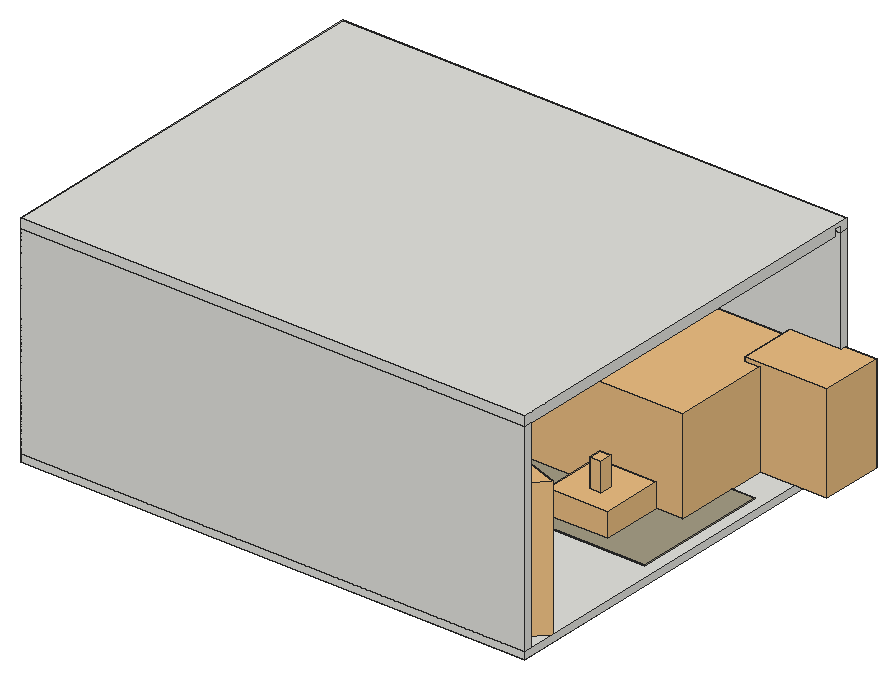
# SketchUp Ruby script. Lengths in inches.
U = 1.inch
M = Sketchup.active_model
def pt(a) = Geom::Point3d.new(a.map { |v| v * U })
def face(e, loops, mat)
  f = e.add_face(loops[0].map { |a| pt(a) })
  loops[1..].each { |l| e.add_face(l.map { |a| pt(a) }).erase! }
  f.material = f.back_material = mat if mat
  f
end
# faces: each face lists its corners as indices into pts; further lists are holes
def faces(e, pts, list, mat = nil) = list.each { |f| face(e, (f[0].is_a?(Array) ? f : [f]).map { |l| l.map { |i| pts[i] } }, mat) }
# xy, xz, yz: faces in a plane at the given z, y or x. An outline is a flat list of corners, or four numbers for a rectangle; further outlines are holes
def ring(l) = l.size == 4 ? [[l[0], l[1]], [l[2], l[1]], [l[2], l[3]], [l[0], l[3]]] : l.each_slice(2).to_a
def flat(e, list, mat, &to3) = list.each { |f| face(e, (f[0].is_a?(Array) ? f : [f]).map { |l| ring(l).map { |u, v| to3.(u, v) } }, mat) }
def xy(e, z, list, mat = nil) = flat(e, list, mat) { |x, y| [x, y, z] }
def xz(e, y, list, mat = nil) = flat(e, list, mat) { |x, z| [x, y, z] }
def yz(e, x, list, mat = nil) = flat(e, list, mat) { |y, z| [x, y, z] }
def lines(e, pts, list) = list.each { |a, b| e.add_line(pt(pts[a]), pt(pts[b])) }
# prism: a flat outline (further loops are holes) pulled along v
def prism(e, loops, v, mat = nil)
  f = face(e, loops, mat); d = Geom::Vector3d.new(v.map { |x| x * U })
  f.pushpull(f.normal.samedirection?(d) ? d.length : -d.length)
end
def box(e, o, s, mat = nil) = prism(e, [[o, [o[0] + s[0], o[1], o[2]], [o[0] + s[0], o[1] + s[1], o[2]], [o[0], o[1] + s[1], o[2]]]], [0, 0, s[2]], mat)
def at(x, y, z, deg = 0) = Geom::Transformation.translation(pt([x, y, z])) * Geom::Transformation.rotation(ORIGIN, Z_AXIS, deg.degrees)
def axes(o, x, y, z) = Geom::Transformation.new([*x, 0, *y, 0, *z, 0, *pt(o).to_a, 1])
def part(name) = M.definitions.add(name)
# library, detail: a bought-in or finely detailed component or shape, given as its bounding box
def library(name, o, s) = part(name).tap { |d| box(d.entities, o, s) }
def detail(e, o, s) = box(e.add_group.entities, o, s)
def put(e, d, t, mat = nil) = e.add_instance(d, t).tap { |i| i.material = mat if mat }
def group(e, t, mat = nil) = e.add_group.tap { |g| g.transformation = t; g.material = mat if mat }.entities
root = M.entities
M.materials.add("Carpet").color = [165, 157, 133]
M.materials.add("Glazing").color = [128, 128, 128]
M.materials["Glazing"].alpha = 0.05
M.materials.add("Powdercoating").color = [41, 44, 40]
c1 = part("Group\#15")
xy(c1.entities,0,[[0,-55.94,0.71,45.94]])
xy(c1.entities,0.2,[[0,-55.94,0.47,45.94],[0.47,45.94,0.71,46.42]])
xy(c1.entities,2.36,[[0.47,-55.94,0.71,46.42]])
xz(c1.entities,-55.94,[[0,0,0.71,0,0.71,2.36,0.47,2.36,0.47,0.2,0,0.2]])
xz(c1.entities,45.94,[[0,0,0.71,0.2]])
xz(c1.entities,46.42,[[0.47,0.2,0.71,2.36]])
yz(c1.entities,0,[[-55.94,0,45.94,0.2]])
yz(c1.entities,0.47,[[-55.94,0.2,46.42,2.36]])
yz(c1.entities,0.71,[[-55.94,0,45.94,0,45.94,0.2,46.42,0.2,46.42,2.36,-55.94,2.36]])
c2 = part("Group\#11")
xy(c2.entities,0,[[0,-59.09,0.71,45.94]])
xy(c2.entities,0.2,[[0,-59.09,0.47,45.94],[0.47,45.94,0.71,46.42]])
xy(c2.entities,2.36,[[0.47,-59.09,0.71,46.42]])
xz(c2.entities,-59.09,[[0,0,0.71,0,0.71,2.36,0.47,2.36,0.47,0.2,0,0.2]])
xz(c2.entities,45.94,[[0,0,0.71,0.2]])
xz(c2.entities,46.42,[[0.47,0.2,0.71,2.36]])
yz(c2.entities,0,[[-59.09,0,45.94,0.2]])
yz(c2.entities,0.47,[[-59.09,0.2,46.42,2.36]])
yz(c2.entities,0.71,[[-59.09,0,45.94,0,45.94,0.2,46.42,0.2,46.42,2.36,-59.09,2.36]])
c3 = part("Group\#16")
prism(c3.entities,[[[0.47,-56.18,0.2],[0,-56.18,0.2],[0,-56.18,0],[0.71,-56.18,0],[0.71,-56.18,2.36],[0.47,-56.18,2.36]]],[0,28.68,0])
c4 = part("Group\#12")
box(c4.entities,[-0.73,0,0],[27.99,0.55,102.05])
c5 = part("Group\#18")
xy(c5.entities,0,[[0.47,-56.18,0.47,-55.47,0,-55.47,0,-28.21,1.18,-28.21,1.18,-56.18]])
xy(c5.entities,0.2,[[0.71,-56.18,1.18,-28.21],[0,-55.47,0.47,-28.21],[0.47,-28.21,0.71,-27.74]])
xy(c5.entities,2.36,[[0.47,-56.18,0.71,-27.74]])
xz(c5.entities,-56.18,[[0.47,0,1.18,0,1.18,0.2,0.71,0.2,0.71,2.36,0.47,2.36]])
xz(c5.entities,-55.47,[[0,0,0.47,0.2]])
xz(c5.entities,-28.21,[[0,0,1.18,0.2]])
xz(c5.entities,-27.74,[[0.47,0.2,0.71,2.36]])
yz(c5.entities,0,[[-55.47,0,-28.21,0.2]])
yz(c5.entities,0.47,[[-56.18,0,-55.47,0.2],[-56.18,0.2,-27.74,2.36]])
yz(c5.entities,0.71,[[-56.18,0.2,-27.74,2.36]])
yz(c5.entities,1.18,[[-56.18,0,-28.21,0.2]])
c6 = part("Group\#34")
xy(c6.entities,0,[[-20.45,0,7.76,1.22]])
xy(c6.entities,0.06,[[-20.39,0.06,7.7,1.22]])
xy(c6.entities,0.47,[[-19.98,0,7.28,0.06]])
xy(c6.entities,101.89,[[-19.98,0,7.28,0.06]])
xy(c6.entities,102.3,[[-20.39,0.06,7.7,1.22]])
xy(c6.entities,102.36,[[-20.45,0,7.76,1.22]])
xz(c6.entities,0,[[[-20.45,0,7.76,102.36],[-19.98,0.47,7.28,101.89]]])
xz(c6.entities,0.06,[[[-20.39,0.06,7.7,102.3],[-19.98,0.47,7.28,101.89]]])
xz(c6.entities,1.22,[[[-20.45,0,7.76,102.36],[-20.39,0.06,7.7,102.3]]])
yz(c6.entities,-20.45,[[0,0,1.22,102.36]])
yz(c6.entities,-20.39,[[0.06,0.06,1.22,102.3]])
yz(c6.entities,-19.98,[[0,0.47,0.06,101.89]])
yz(c6.entities,7.28,[[0,0.47,0.06,101.89]])
yz(c6.entities,7.7,[[0.06,0.06,1.22,102.3]])
yz(c6.entities,7.76,[[0,0,1.22,102.36]])
c7 = part("Group\#14")
put(c7.entities,c1,axes([27.97,0,7.875],[1,0,0],[0,0,-1],[0,1,0]),"Powdercoating")
put(c7.entities,c2,axes([0.71,0,6.8],[-1,0,0],[0,0,-0.97687],[0,1,0]),"Powdercoating")
put(c7.entities,c3,axes([-27.5,0,-38.07],[0,0,-1],[-1,0,0],[0,1,0]),"Powdercoating")
put(c7.entities,c4,at(1.12,0.35,-38.39),"Glazing")
put(c7.entities,c5,axes([-27.5,0,63.35],[0,0,1],[-1,0,0],[0,1,0]),"Powdercoating")
put(c7.entities,c6,at(20.6875,1.0625,-38.54),"Powdercoating")
c8 = part("Sliding door panels")
put(c8.entities,c7,at(-1.18,4.5,38.86))
g1 = group(c8.entities,at(84.74,4.5,38.86))
put(g1,c1,axes([-27.97,0,7.875],[-1,0,0],[0,0,-1],[0,1,0]),"Powdercoating")
put(g1,c2,axes([-0.71,0,6.8],[1,0,0],[0,0,-0.97687],[0,1,0]),"Powdercoating")
put(g1,c3,axes([27.5,0,-38.07],[0,0,-1],[1,0,0],[0,1,0]),"Powdercoating")
put(g1,c4,axes([-1.12,0.35,-38.39],[-1,0,0],[0,1,0],[0,0,1]),"Glazing")
put(g1,c5,axes([27.5,0,63.35],[0,0,1],[1,0,0],[0,1,0]),"Powdercoating")
put(g1,c6,axes([-20.6875,1.0625,-38.54],[-1,0,0],[0,1,0],[0,0,1]),"Powdercoating")
g2 = group(c8.entities,at(56.0625,4.5,38.86))
put(g2,c1,axes([-27.97,0,7.875],[-1,0,0],[0,0,-1],[0,1,0]),"Powdercoating")
put(g2,c3,axes([27.5,0,-38.07],[0,0,-1],[1,0,0],[0,1,0]),"Powdercoating")
put(g2,c4,axes([-1.12,0.35,-38.39],[-1,0,0],[0,1,0],[0,0,1]),"Glazing")
put(g2,c5,axes([27.5,0,63.35],[0,0,1],[1,0,0],[0,1,0]),"Powdercoating")
put(g2,c6,axes([-20.6875,1.0625,-38.54],[-1,0,0],[0,1,0],[0,0,1]),"Powdercoating")
g3 = group(g2,at(-0.71,0,6.8),"Powdercoating")
xy(g3,-45.34,[[0.47,0.2,0.71,2.36]])
xy(g3,-44.88,[[0,0,0.71,0.2]])
xy(g3,57.73,[[0,0,0.71,0,0.71,2.36,0.47,2.36,0.47,0.2,0,0.2]])
xz(g3,0,[[0,-44.88,0.71,57.73]])
xz(g3,0.2,[[0.47,-45.34,0.71,-44.88],[0,-44.88,0.47,57.73]])
xz(g3,2.36,[[0.47,-45.34,0.71,57.73]])
yz(g3,0,[[0,-44.88,0.2,57.73]])
yz(g3,0.47,[[0.2,-45.34,2.36,57.73]])
yz(g3,0.71,[[0.2,-45.34,2.36,-45.34,2.36,57.73,0,57.73,0,-44.88,0.2,-44.88]])
put(c8.entities,c7,axes([-33.94,4.5,38.86],[1.14218,0,0],[0,1,0],[0,0,1]))
c9 = part("sliding door")
put(c9.entities,c8,at(0,-4.5,-0.08))
c10 = library("____",[-857.35,-17.89,-0.54],[1669.93,232.85,2261.28])
c11 = library("_________4",[391.51,-229.42,0.9375],[996.96,302.79,2265.625])
c12 = library("_________5\#1",[-1361.6,-221.02,-25.09],[914.12,296.77,2295.03])
c13 = library("door58",[0,0,0],[34.0625,4.69,78.29])
c14 = library("Sectional sofa",[-0.93,-10.63,-23.92],[126.92,88.46,78.25])
c15 = part("Vertical bar")
box(c15.entities,[0,0,0],[0.875,0.8,31.5])
c16 = library("skpE45D",[-24.47,-26.97,0],[48.94,53.94,77.79])
c17 = part("Tapete")
box(c17.entities,[0,0,0],[73.55,109.57,0.42],"Carpet")
c18 = part("02 Tapete")
put(c18.entities,c17,at(0.05,-109.34,0))
c19 = part("Carpet")
put(c19.entities,c18,at(0,0,0))
c20 = library("Round Coffe Table",[-17.98,-18.01,-0.01],[35.96,36.02,14.19])
c21 = library("191418",[-24.78,-19.8125,0],[49.1,36.6,58.24])
c22 = library("Flower Vase",[5.42,3.34,0],[6.62,7.58,17.36])
c23 = part("Component\#6")
xy(c23.entities,0,[[[1.86,0,1.34,0.1,0.88,0.34,0.49,0.68,0.2,1.12,0.03,1.61,0,2.13,0.1,2.65,0.34,3.11,0.68,3.5,1.12,3.79,1.61,3.96,2.13,3.99,2.65,3.89,3.11,3.65,3.5,3.31,3.79,2.87,3.96,2.38,3.99,1.86,3.89,1.34,3.65,0.88,3.31,0.49,2.87,0.2,2.38,0.03],[1.9,0.61,2.26,0.64,2.6,0.75,2.9,0.95,3.14,1.22,3.3,1.54,3.375,1.9,3.35,2.26,3.24,2.6,3.04,2.9,2.77,3.14,2.45,3.3,2.09,3.375,1.73,3.35,1.39,3.24,1.09,3.04,0.85,2.77,0.6875,2.45,0.61,2.09,0.64,1.73,0.75,1.39,0.95,1.09,1.22,0.85,1.54,0.6875]]])
xy(c23.entities,0.125,[[1.9,0.61,1.54,0.6875,1.22,0.85,0.95,1.09,0.75,1.39,0.64,1.73,0.61,2.09,0.6875,2.45,0.85,2.77,1.09,3.04,1.39,3.24,1.73,3.35,2.09,3.375,2.45,3.3,2.77,3.14,3.04,2.9,3.24,2.6,3.35,2.26,3.375,1.9,3.3,1.54,3.14,1.22,2.9,0.95,2.6,0.75,2.26,0.64]])
xy(c23.entities,0.75,[[1.86,0,2.38,0.03,2.87,0.2,3.31,0.49,3.65,0.88,3.89,1.34,3.99,1.86,3.96,2.38,3.79,2.87,3.5,3.31,3.11,3.65,2.65,3.89,2.13,3.99,1.61,3.96,1.12,3.79,0.68,3.5,0.34,3.11,0.1,2.65,0,2.13,0.03,1.61,0.2,1.12,0.49,0.68,0.88,0.34,1.34,0.1]])
p = [[1.34,0.1,0],[1.86,0,0],[1.86,0,0.75],[1.34,0.1,0.75],[2.38,0.03,0],[2.38,0.03,0.75],
  [2.87,0.2,0],[2.87,0.2,0.75],[0.88,0.34,0],[0.88,0.34,0.75],[3.31,0.49,0],[3.31,0.49,0.75],
  [0.49,0.68,0],[0.49,0.68,0.75],[3.65,0.88,0],[3.65,0.88,0.75],[1.9,0.61,0],[1.54,0.6875,0],
  [1.54,0.6875,0.125],[1.9,0.61,0.125],[2.26,0.64,0],[2.26,0.64,0.125],[2.6,0.75,0],[2.6,0.75,0.125],
  [0.2,1.12,0],[0.2,1.12,0.75],[1.22,0.85,0],[1.22,0.85,0.125],[0.95,1.09,0],[0.95,1.09,0.125],
  [2.9,0.95,0],[2.9,0.95,0.125],[3.89,1.34,0],[3.89,1.34,0.75],[3.14,1.22,0],[3.14,1.22,0.125],
  [0.03,1.61,0],[0.03,1.61,0.75],[0.75,1.39,0],[0.75,1.39,0.125],[3.3,1.54,0],[3.3,1.54,0.125],
  [3.99,1.86,0],[3.99,1.86,0.75],[0.64,1.73,0],[0.64,1.73,0.125],[3.375,1.9,0],[3.375,1.9,0.125],
  [0,2.13,0],[0,2.13,0.75],[0.61,2.09,0],[0.61,2.09,0.125],[3.35,2.26,0],[3.35,2.26,0.125],
  [3.96,2.38,0],[3.96,2.38,0.75],[0.1,2.65,0],[0.1,2.65,0.75],[0.6875,2.45,0],[0.6875,2.45,0.125],
  [3.24,2.6,0],[3.24,2.6,0.125],[0.85,2.77,0],[0.85,2.77,0.125],[3.79,2.87,0],[3.79,2.87,0.75],
  [0.34,3.11,0],[0.34,3.11,0.75],[3.04,2.9,0],[3.04,2.9,0.125],[1.09,3.04,0],[1.09,3.04,0.125],
  [2.77,3.14,0],[2.77,3.14,0.125],[3.5,3.31,0],[3.5,3.31,0.75],[1.39,3.24,0],[1.39,3.24,0.125],
  [0.68,3.5,0],[0.68,3.5,0.75],[2.45,3.3,0],[2.45,3.3,0.125],[1.73,3.35,0],[1.73,3.35,0.125],
  [2.09,3.375,0],[2.09,3.375,0.125],[3.11,3.65,0],[3.11,3.65,0.75],[1.12,3.79,0],[1.12,3.79,0.75],
  [2.65,3.89,0],[2.65,3.89,0.75],[1.61,3.96,0],[1.61,3.96,0.75],[2.13,3.99,0],[2.13,3.99,0.75]]
faces(c23.entities,p,[[0,1,2,3],[1,4,5,2],[4,6,7,5],[8,0,3,9],[6,10,11,7],[12,8,9,13],[10,14,15,11],[16,17,18,19],
  [20,16,19,21],[22,20,21,23],[24,12,13,25],[17,26,27,18],[26,28,29,27],[30,22,23,31],[14,32,33,15],[34,30,31,35],
  [36,24,25,37],[28,38,39,29],[40,34,35,41],[32,42,43,33],[38,44,45,39],[46,40,41,47],[48,36,37,49],[44,50,51,45],
  [52,46,47,53],[42,54,55,43],[56,48,49,57],[50,58,59,51],[60,52,53,61],[58,62,63,59],[54,64,65,55],[66,56,57,67],
  [68,60,61,69],[62,70,71,63],[72,68,69,73],[64,74,75,65],[70,76,77,71],[78,66,67,79],[80,72,73,81],[76,82,83,77],
  [84,80,81,85],[74,86,87,75],[82,84,85,83],[88,78,79,89],[86,90,91,87],[92,88,89,93],[90,94,95,91],[94,92,93,95]])
c24 = library("VASE ",[-5.43,-0.85,0],[32.15,30.91,75.86])
c25 = part("Group30\#1")
p = [[30,30,37],[124.5,30,37],[30,115.5,37]]
lines(c25.entities,p,[[0,1],[0,2]])
c26 = part("Group29\#1")
put(c26.entities,c25,at(0,0,0))
c27 = part("Group\#40")
box(c27.entities,[0,0,87.15],[0.75,23.85,29.85])
xy(c27.entities,0,[[0,0,0.75,23.85]])
xy(c27.entities,14.11,[[0.25,0.25,0.75,23.6]])
xy(c27.entities,14.61,[[0.25,0.25,0.75,23.6]])
xy(c27.entities,14.86,[[0,0,0.75,23.85]])
xy(c27.entities,15.16,[[0,0,0.75,23.85]])
xy(c27.entities,29.26,[[0.25,0.25,0.75,23.6]])
xy(c27.entities,29.76,[[0.25,0.25,0.75,23.6]])
xy(c27.entities,30.01,[[0,0,0.75,23.85]])
xy(c27.entities,30.3125,[[0,0,0.75,23.85]])
xy(c27.entities,86.85,[[0,0,0.75,23.85]])
xz(c27.entities,0,[[0,0,0.75,14.86],[0,15.16,0.75,30.01],[0,30.3125,0.75,86.85]])
xz(c27.entities,0.25,[[0.25,14.11,0.75,14.61],[0.25,29.26,0.75,29.76]])
xz(c27.entities,23.6,[[0.25,14.11,0.75,14.61],[0.25,29.26,0.75,29.76]])
xz(c27.entities,23.85,[[0,0,0.75,14.86],[0,15.16,0.75,30.01],[0,30.3125,0.75,86.85]])
yz(c27.entities,0,[[0,0,23.85,14.86],[0,14.86,23.85,15.16],[0,15.16,23.85,30.01],[0,30.01,23.85,30.3125],[0,30.3125,23.85,86.85]])
yz(c27.entities,0.25,[[0.25,14.11,23.6,14.61],[0.25,29.26,23.6,29.76]])
yz(c27.entities,0.75,[[0,0,23.85,13.86],[[0,13.86,23.85,14.86],[0.25,14.11,23.6,14.61]],[0,15.16,23.85,29.01],[[0,29.01,23.85,30.01],[0.25,29.26,23.6,29.76]],[0,30.3125,23.85,86.85]])
p = [[0,0,86.85],[0,0,87.15],[0,23.85,86.85],[0,23.85,87.15]]
lines(c27.entities,p,[[0,1],[2,3]])
c28 = library("Agrupar\#9",[0,0,0],[23.62,23.23,23.62])
c29 = library("Group\#41",[0,0,-0.5],[89.46,0.75,39.5])
c30 = library("Group\#39",[0,0,0],[23.23,23.62,41.34])
c31 = library("Group\#38",[0,0,-0.5],[59.03,0.75,39.5])
c32 = library("Group\#45",[0,0,0],[67.25,19.4,51.93])
c33 = library("Groupe\#5",[0,0,0],[91.34,77.95,241.79])
c34 = library("Group\#46",[0,0,0],[2,2,36.3125])
p = [[17,36.7,61],[17,56.25,61],[17,76.1,61],[17,95.8,61]]
lines(root,p,[[0,1],[1,2],[2,3]])
put(root,c9,axes([69.57,235.5,4],[1.21,0,0],[0,1.4525,0],[0,0,1.04543]))
put(root,c10,axes([33.86,232,4.15],[0.01804,0,0],[0,0.02091,0],[0,0,0.05412]))
put(root,c11,axes([140.46,233.33,5.36],[0.03072,0,0],[0,0.01858,0],[0,0,0.05359]))
put(root,c12,axes([29.18,233.52,5.36],[0.01813,0,0],[0,0.01598,0],[0,0,0.05359]))
put(root,c10,axes([149.23,232,4.15],[0.01263,0,0],[0,0.02091,0],[0,0,0.05412]))
put(root,c13,axes([0,229.5,4],[0,-1.233,0],[1.05479,0,0],[0,0,1.07289]))
put(root,c14,at(277.88,222.27,5.63,-180))
put(root,c15,at(106,90,4))
put(root,c15,at(106,91.1875,4))
put(root,c15,at(106,92.38,4))
put(root,c15,at(106,93.57,4))
put(root,c15,at(106,94.76,4))
put(root,c15,at(106,95.95,4))
put(root,c15,at(106,97.14,4))
put(root,c15,at(106,98.33,4))
put(root,c15,at(106,99.51,4))
put(root,c15,at(106,100.7,4))
put(root,c15,at(106,101.89,4))
put(root,c15,at(106,103.08,4))
put(root,c15,at(106,104.27,4))
put(root,c15,at(106,105.46,4))
put(root,c15,at(106,106.65,4))
put(root,c15,at(106,107.84,4))
put(root,c15,at(106,109.03,4))
put(root,c15,at(106,110.22,4))
put(root,c15,at(106,111.41,4))
put(root,c15,at(106,112.6,4))
put(root,c15,at(106,113.79,4))
put(root,c15,at(106,114.98,4))
put(root,c15,at(106,116.17,4))
put(root,c15,at(106,117.36,4))
put(root,c15,at(106,118.54,4))
put(root,c15,at(106,119.73,4))
put(root,c15,at(106,120.92,4))
put(root,c15,at(106,122.11,4))
put(root,c15,at(106,123.3,4))
put(root,c15,at(106,124.49,4))
put(root,c15,at(106,125.68,4))
put(root,c15,at(106,126.87,4))
put(root,c15,at(106,128.06,4))
put(root,c15,at(106,129.25,4))
put(root,c15,at(106,130.4375,4))
put(root,c15,at(106,131.63,4))
put(root,c15,at(106,132.82,4))
put(root,c15,at(106,134.01,4))
put(root,c15,at(106,135.2,4))
put(root,c15,at(106,136.39,4))
put(root,c15,at(106,137.57,4))
put(root,c15,at(106,138.76,4))
put(root,c15,at(106,139.95,4))
put(root,c15,at(106,141.14,4))
put(root,c15,at(106,142.33,4))
put(root,c15,at(106,143.52,4))
put(root,c15,at(106,144.71,4))
put(root,c15,at(106,145.9,4))
put(root,c15,at(106,147.09,4))
put(root,c15,at(106,148.28,4))
put(root,c15,at(106,149.47,4))
put(root,c15,at(106,150.66,4))
put(root,c15,at(106,151.85,4))
put(root,c15,at(106,153.04,4))
put(root,c15,at(106,154.23,4))
put(root,c15,at(106,155.41,4))
put(root,c15,at(106,156.6,4))
put(root,c15,at(106,157.79,4))
put(root,c15,at(106,158.98,4))
put(root,c15,at(106,160.17,4))
put(root,c15,at(106,161.36,4))
put(root,c15,at(106,162.55,4))
put(root,c15,at(106,163.74,4))
put(root,c15,at(106,164.93,4))
put(root,c15,at(106,166.12,4))
put(root,c15,at(106,167.31,4))
put(root,c15,at(106,168.5,4))
put(root,c15,at(106,169.6875,4))
put(root,c15,at(106,170.875,4))
put(root,c15,at(106,172.07,4))
put(root,c15,at(106,173.26,4))
put(root,c15,at(106,174.44,4))
put(root,c15,at(106,175.63,4))
put(root,c15,at(106,176.82,4))
put(root,c15,at(106,178.01,4))
put(root,c15,at(106,179.2,4))
put(root,c16,axes([118.4,107.06,4],[0,-0.352,0],[0.348,0,0],[0,0,0.40001]))
put(root,c16,axes([118.4,163.19,4],[0,-0.352,0],[0.348,0,0],[0,0,0.40001]))
put(root,c19,axes([292.68,180.45,4],[0,-1.11,0],[1.12,0,0],[0,0,1]))
put(root,c16,axes([118.4,134.94,4],[0,-0.352,0],[0.348,0,0],[0,0,0.40001]))
put(root,c20,at(245.5,125.8,4.42))
put(root,c21,at(294.53,221.51,4))
put(root,c22,at(237.44,116.68,17.73))
put(root,c23,at(55.62,44.18,123.25))
put(root,c23,at(55.62,91.06,123.25))
put(root,c23,at(55.62,142.31,123.25))
put(root,c23,at(55.62,186.87,123.25))
put(root,c23,at(132.3,142.31,123.25))
put(root,c23,at(132.3,186.87,123.25))
put(root,c23,at(132.3,44.18,123.25))
put(root,c23,at(132.3,91.06,123.25))
put(root,c24,axes([91.33,92.08,37],[0.56,0,0],[0,0.52,0],[0,0,0.31638]))
g4 = group(root,at(0,0,0))
box(g4,[0,0,0],[300,240,4])
g5 = group(root,at(0,0,4))
box(g5,[0,0,0],[300,4.5,120])
g6 = group(root,at(0,235.5,4))
prism(g6,[[[300,4.5,0],[172.5,4.5,0],[172.5,4.5,108],[28.5,4.5,108],[28.5,4.5,0],[0,4.5,0],[0,4.5,120],[300,4.5,120]]],[0,-4.5,0])
g7 = group(root,at(0,4.5,4))
xy(g7,0,[[0,0,4.5,183],[0,225,4.5,231]])
xy(g7,84,[[0,183,4.5,225]])
xy(g7,120,[[0,0,4.5,231]])
xz(g7,0,[[0,0,4.5,120]])
xz(g7,183,[[0,0,4.5,84]])
xz(g7,225,[[0,0,4.5,84]])
xz(g7,231,[[0,0,4.5,120]])
yz(g7,0,[[0,0,0,120,231,120,231,0,225,0,225,84,183,84,183,0]])
yz(g7,4.5,[[0,0,183,0,183,84,225,84,225,0,231,0,231,120,0,120]])
p = [[4.5,177,84],[4.5,177,120]]
lines(g7,p,[[0,1]])
g8 = group(root,at(4.5,4.5,4))
xy(g8,0,[[0,0,0,111,23.5,111,23.5,24,120,24,120,0]])
xy(g8,3,[[23.5,24,24,111]])
xy(g8,31.5,[[24,24,24,25,25,25,25,25.5,120,25.5,120,24],[24,25,24,111,25.5,111,25.5,25.5,25,25.5,25,25]])
xy(g8,33,[[0,0,120,0,120,25.5,25.5,25.5,25.5,111,0,111]])
xz(g8,0,[[0,0,120,33]])
xz(g8,24,[[23.5,0,120,3],[24,3,120,31.5]])
xz(g8,25.5,[[25.5,31.5,120,33]])
xz(g8,111,[[0,0,0,33,25.5,33,25.5,31.5,24,31.5,24,3,23.5,3,23.5,0]])
yz(g8,0,[[0,0,111,33]])
yz(g8,23.5,[[24,0,111,3]])
yz(g8,24,[[24,3,111,31.5]])
yz(g8,25.5,[[25.5,31.5,111,33]])
yz(g8,120,[[0,0,24,0,24,31.5,25.5,31.5,25.5,33,0,33]])
g9 = group(g8,at(40.15,24,3))
xy(g9,0,[[-16.15,0,-0.45,0.75],[0,0,15.7,0.75],[16,0,31.7,0.75],[32,0,47.7,0.75],[48,0,63.7,0.75],
  [64,0,79.85,0.75]])
xy(g9,8.6,[[16.25,0.4375,31.45,0.75],[32.25,0.4375,47.45,0.75]])
xy(g9,9.1,[[16.25,0.4375,31.45,0.75],[32.25,0.4375,47.45,0.75]])
xy(g9,9.35,[[16,0,31.7,0.75],[32,0,47.7,0.75]])
xy(g9,9.65,[[16,0,31.7,0.75],[32,0,47.7,0.75]])
xy(g9,18.1,[[16.25,0.4375,31.45,0.75],[32.25,0.4375,47.45,0.75]])
xy(g9,18.6,[[16.25,0.4375,31.45,0.75],[32.25,0.4375,47.45,0.75]])
xy(g9,18.85,[[16,0,31.7,0.75],[32,0,47.7,0.75]])
xy(g9,19.15,[[16,0,31.7,0.75],[32,0,47.7,0.75]])
xy(g9,27.75,[[-15.9,0.4375,-0.7,0.75],[0.25,0.4375,15.45,0.75],[16.25,0.4375,31.45,0.75],[32.25,0.4375,47.45,0.75],[48.25,0.4375,63.45,0.75]])
xy(g9,28.25,[[-15.9,0.4375,-0.7,0.75],[0.25,0.4375,15.45,0.75],[16.25,0.4375,31.45,0.75],[32.25,0.4375,47.45,0.75],[48.25,0.4375,63.45,0.75]])
xy(g9,28.5,[[-16.15,0,-0.45,0.75],[0,0,15.7,0.75],[16,0,31.7,0.75],[32,0,47.7,0.75],[48,0,63.7,0.75],
  [64,0,79.85,0.75]])
xz(g9,0,[[-16.15,0,-0.45,28.5],[0,0,15.7,28.5],[16,0,31.7,9.35],[32,0,47.7,9.35],[48,0,63.7,28.5],
  [64,0,79.85,28.5],[16,9.35,31.7,9.65],[32,9.35,47.7,9.65],[16,9.65,31.7,18.85],[32,9.65,47.7,18.85],
  [16,18.85,31.7,19.15],[32,18.85,47.7,19.15],[16,19.15,31.7,28.5],[32,19.15,47.7,28.5]])
xz(g9,0.4375,[[16.25,8.6,31.45,9.1],[32.25,8.6,47.45,9.1],[16.25,18.1,31.45,18.6],[32.25,18.1,47.45,18.6],[-15.9,27.75,-0.7,28.25],
  [0.25,27.75,15.45,28.25],[16.25,27.75,31.45,28.25],[32.25,27.75,47.45,28.25],[48.25,27.75,63.45,28.25]])
xz(g9,0.75,[[-16.15,0,-0.45,27.5],[0,0,15.7,27.5],[16,0,31.7,8.35],[32,0,47.7,8.35],[48,0,63.7,27.5],
  [64,0,79.85,27.5],[[16,8.35,31.7,9.35],[16.25,8.6,31.45,9.1]],[[32,8.35,47.7,9.35],[32.25,8.6,47.45,9.1]],[16,9.65,31.7,17.85],[32,9.65,47.7,17.85],
  [[16,17.85,31.7,18.85],[16.25,18.1,31.45,18.6]],[[32,17.85,47.7,18.85],[32.25,18.1,47.45,18.6]],[16,19.15,31.7,27.5],[32,19.15,47.7,27.5],[[-16.15,27.5,-0.45,28.5],[-15.9,27.75,-0.7,28.25]],
  [[0,27.5,15.7,28.5],[0.25,27.75,15.45,28.25]],[[16,27.5,31.7,28.5],[16.25,27.75,31.45,28.25]],[[32,27.5,47.7,28.5],[32.25,27.75,47.45,28.25]],[[48,27.5,63.7,28.5],[48.25,27.75,63.45,28.25]],[[64,27.5,79.85,28.5],[64.25,27.75,79.6,28.25]],
  [64.25,27.75,79.6,28.25]])
yz(g9,-16.15,[[0,0,0.75,28.5]])
yz(g9,-15.9,[[0.4375,27.75,0.75,28.25]])
yz(g9,-0.7,[[0.4375,27.75,0.75,28.25]])
yz(g9,-0.45,[[0,0,0.75,28.5]])
yz(g9,0,[[0,0,0.75,28.5]])
yz(g9,0.25,[[0.4375,27.75,0.75,28.25]])
yz(g9,15.45,[[0.4375,27.75,0.75,28.25]])
yz(g9,15.7,[[0,0,0.75,28.5]])
yz(g9,16,[[0,0,0.75,9.35],[0,9.65,0.75,18.85],[0,19.15,0.75,28.5]])
yz(g9,16.25,[[0.4375,8.6,0.75,9.1],[0.4375,18.1,0.75,18.6],[0.4375,27.75,0.75,28.25]])
yz(g9,31.45,[[0.4375,8.6,0.75,9.1],[0.4375,18.1,0.75,18.6],[0.4375,27.75,0.75,28.25]])
yz(g9,31.7,[[0,0,0.75,9.35],[0,9.65,0.75,18.85],[0,19.15,0.75,28.5]])
yz(g9,32,[[0,0,0.75,9.35],[0,9.65,0.75,18.85],[0,19.15,0.75,28.5]])
yz(g9,32.25,[[0.4375,8.6,0.75,9.1],[0.4375,18.1,0.75,18.6],[0.4375,27.75,0.75,28.25]])
yz(g9,47.45,[[0.4375,8.6,0.75,9.1],[0.4375,18.1,0.75,18.6],[0.4375,27.75,0.75,28.25]])
yz(g9,47.7,[[0,0,0.75,9.35],[0,9.65,0.75,18.85],[0,19.15,0.75,28.5]])
yz(g9,48,[[0,0,0.75,28.5]])
yz(g9,48.25,[[0.4375,27.75,0.75,28.25]])
yz(g9,63.45,[[0.4375,27.75,0.75,28.25]])
yz(g9,63.7,[[0,0,0.75,28.5]])
yz(g9,64,[[0,0,0.75,28.5]])
yz(g9,79.85,[[0,0,0.75,28.5]])
put(g8,c26,at(-4.5,-4.5,-4))
g10 = group(g8,at(28.5,94.79,3,-90))
xy(g10,0,[[-16.11,-4.5,-0.41,-3.75],[-0.11,-4.5,15.9,-3.75],[16.04,-4.5,34.88,-3.75],[35.24,-4.5,54.08,-3.75],[54.21,-4.5,69.91,-3.75]])
xy(g10,8.6,[[16.34,-4.0625,34.58,-3.75],[35.54,-4.0625,53.78,-3.75]])
xy(g10,9.1,[[16.34,-4.0625,34.58,-3.75],[35.54,-4.0625,53.78,-3.75]])
xy(g10,9.35,[[16.04,-4.5,34.88,-3.75],[35.24,-4.5,54.08,-3.75]])
xy(g10,9.65,[[16.04,-4.5,34.88,-3.75],[35.24,-4.5,54.08,-3.75]])
xy(g10,18.1,[[16.34,-4.0625,34.58,-3.75],[35.54,-4.0625,53.78,-3.75]])
xy(g10,18.6,[[16.34,-4.0625,34.58,-3.75],[35.54,-4.0625,53.78,-3.75]])
xy(g10,18.85,[[16.04,-4.5,34.88,-3.75],[35.24,-4.5,54.08,-3.75]])
xy(g10,19.15,[[16.04,-4.5,34.88,-3.75],[35.24,-4.5,54.08,-3.75]])
xy(g10,27.75,[[-15.86,-4.0625,-0.66,-3.75],[0.14,-4.0625,15.65,-3.75],[16.34,-4.0625,34.58,-3.75],[35.54,-4.0625,53.78,-3.75],[54.46,-4.0625,69.66,-3.75]])
xy(g10,28.25,[[-15.86,-4.0625,-0.66,-3.75],[0.14,-4.0625,15.65,-3.75],[16.34,-4.0625,34.58,-3.75],[35.54,-4.0625,53.78,-3.75],[54.46,-4.0625,69.66,-3.75]])
xy(g10,28.5,[[-16.11,-4.5,-0.41,-3.75],[-0.11,-4.5,15.9,-3.75],[16.04,-4.5,34.88,-3.75],[35.24,-4.5,54.08,-3.75],[54.21,-4.5,69.91,-3.75]])
xz(g10,-4.5,[[-16.11,0,-0.41,28.5],[-0.11,0,15.9,28.5],[16.04,0,34.88,9.35],[35.24,0,54.08,9.35],[54.21,0,69.91,28.5],
  [16.04,9.35,34.88,9.65],[35.24,9.35,54.08,9.65],[16.04,9.65,34.88,18.85],[35.24,9.65,54.08,18.85],[16.04,18.85,34.88,19.15],
  [35.24,18.85,54.08,19.15],[16.04,19.15,34.88,28.5],[35.24,19.15,54.08,28.5]])
xz(g10,-4.0625,[[16.34,8.6,34.58,9.1],[35.54,8.6,53.78,9.1],[16.34,18.1,34.58,18.6],[35.54,18.1,53.78,18.6],[-15.86,27.75,-0.66,28.25],
  [0.14,27.75,15.65,28.25],[16.34,27.75,34.58,28.25],[35.54,27.75,53.78,28.25],[54.46,27.75,69.66,28.25]])
xz(g10,-3.75,[[-16.11,0,-0.41,27.5],[-0.11,0,15.9,27.5],[16.04,0,34.88,8.35],[35.24,0,54.08,8.35],[54.21,0,69.91,27.5],
  [[16.04,8.35,34.88,9.35],[16.34,8.6,34.58,9.1]],[[35.24,8.35,54.08,9.35],[35.54,8.6,53.78,9.1]],[16.04,9.65,34.88,17.85],[35.24,9.65,54.08,17.85],[[16.04,17.85,34.88,18.85],[16.34,18.1,34.58,18.6]],
  [[35.24,17.85,54.08,18.85],[35.54,18.1,53.78,18.6]],[16.04,19.15,34.88,27.5],[35.24,19.15,54.08,27.5],[[-16.11,27.5,-0.41,28.5],[-15.86,27.75,-0.66,28.25]],[[-0.11,27.5,15.9,28.5],[0.14,27.75,15.65,28.25]],
  [[16.04,27.5,34.88,28.5],[16.34,27.75,34.58,28.25]],[[35.24,27.5,54.08,28.5],[35.54,27.75,53.78,28.25]],[[54.21,27.5,69.91,28.5],[54.46,27.75,69.66,28.25]]])
yz(g10,-16.11,[[-4.5,0,-3.75,28.5]])
yz(g10,-15.86,[[-4.0625,27.75,-3.75,28.25]])
yz(g10,-0.66,[[-4.0625,27.75,-3.75,28.25]])
yz(g10,-0.41,[[-4.5,0,-3.75,28.5]])
yz(g10,-0.11,[[-4.5,0,-3.75,28.5]])
yz(g10,0.14,[[-4.0625,27.75,-3.75,28.25]])
yz(g10,15.65,[[-4.0625,27.75,-3.75,28.25]])
yz(g10,15.9,[[-4.5,0,-3.75,28.5]])
yz(g10,16.04,[[-4.5,0,-3.75,9.35],[-4.5,9.65,-3.75,18.85],[-4.5,19.15,-3.75,28.5]])
yz(g10,16.34,[[-4.0625,8.6,-3.75,9.1],[-4.0625,18.1,-3.75,18.6],[-4.0625,27.75,-3.75,28.25]])
yz(g10,34.58,[[-4.0625,8.6,-3.75,9.1],[-4.0625,18.1,-3.75,18.6],[-4.0625,27.75,-3.75,28.25]])
yz(g10,34.88,[[-4.5,0,-3.75,9.35],[-4.5,9.65,-3.75,18.85],[-4.5,19.15,-3.75,28.5]])
yz(g10,35.24,[[-4.5,0,-3.75,9.35],[-4.5,9.65,-3.75,18.85],[-4.5,19.15,-3.75,28.5]])
yz(g10,35.54,[[-4.0625,8.6,-3.75,9.1],[-4.0625,18.1,-3.75,18.6],[-4.0625,27.75,-3.75,28.25]])
yz(g10,53.78,[[-4.0625,8.6,-3.75,9.1],[-4.0625,18.1,-3.75,18.6],[-4.0625,27.75,-3.75,28.25]])
yz(g10,54.08,[[-4.5,0,-3.75,9.35],[-4.5,9.65,-3.75,18.85],[-4.5,19.15,-3.75,28.5]])
yz(g10,54.21,[[-4.5,0,-3.75,28.5]])
yz(g10,54.46,[[-4.0625,27.75,-3.75,28.25]])
yz(g10,69.66,[[-4.0625,27.75,-3.75,28.25]])
yz(g10,69.91,[[-4.5,0,-3.75,28.5]])
put(root,c27,at(28.5,115.5,7))
g11 = group(root,at(28.5,139.5,7))
xy(g11,0,[[0,0.15,0.75,24]])
xy(g11,14.11,[[0.25,0.4,0.75,23.75]])
xy(g11,14.61,[[0.25,0.4,0.75,23.75]])
xy(g11,14.86,[[0,0.15,0.75,24]])
xy(g11,15.16,[[0,0.15,0.75,24]])
xy(g11,29.26,[[0.25,0.4,0.75,23.75]])
xy(g11,29.76,[[0.25,0.4,0.75,23.75]])
xy(g11,30.01,[[0,0.15,0.75,24]])
xy(g11,30.3125,[[-3.0625,0.15,0,24]])
xy(g11,53.93,[[-3.0625,0.15,0,24]])
xy(g11,53.99,[[0,0.15,0.75,24]])
xy(g11,86.85,[[0,0.15,0.75,24]])
xy(g11,87.15,[[0,0.15,0.75,24]])
xy(g11,117,[[0,0.15,0.75,24]])
xz(g11,0.15,[[0,0,0.75,14.86],[0,15.16,0.75,30.01],[-3.0625,30.3125,0,53.93],[0,53.99,0.75,86.85],[0,87.15,0.75,117]])
xz(g11,0.4,[[0.25,14.11,0.75,14.61],[0.25,29.26,0.75,29.76]])
xz(g11,23.75,[[0.25,14.11,0.75,14.61],[0.25,29.26,0.75,29.76]])
xz(g11,24,[[0,0,0.75,14.86],[0,15.16,0.75,30.01],[-3.0625,30.3125,0,53.93],[0,53.99,0.75,86.85],[0,87.15,0.75,117]])
yz(g11,0,[[0.15,0,24,14.86],[0.15,14.86,24,15.16],[0.15,15.16,24,30.01],[0.15,30.01,24,30.3125],[0.15,53.93,24,53.99],
  [0.15,53.99,24,86.85],[0.15,86.85,24,87.15],[0.15,87.15,24,117]])
yz(g11,0.25,[[0.4,14.11,23.75,14.61],[0.4,29.26,23.75,29.76]])
yz(g11,0.75,[[0.15,0,24,13.86],[[0.15,13.86,24,14.86],[0.4,14.11,23.75,14.61]],[0.15,15.16,24,29.01],[[0.15,29.01,24,30.01],[0.4,29.26,23.75,29.76]],[0.15,53.99,24,86.85],
  [0.15,87.15,24,117]])
g12 = group(root,at(4.5,115.5,4))
xy(g12,0,[[0,0,23.5,66]])
xy(g12,3,[[23.5,0,24,24],[23.5,24,24,48],[23.5,48,24,66]])
xy(g12,3.5,[[0.5,48.5,24,65.5]])
xy(g12,26.45,[[0.5,48.5,24,65.5]])
xy(g12,26.95,[[0.5,48.5,24,65.5]])
xy(g12,33.3125,[[0.5,24.15,24,48]])
xy(g12,49.65,[[0.5,48.5,24,65.5]])
xy(g12,50.15,[[0.5,48.5,24,65.5]])
xy(g12,56.93,[[0.5,24.15,24,48]])
xy(g12,72.85,[[0.5,48.5,24,65.5]])
xy(g12,73.35,[[0.5,48.5,24,65.5]])
xy(g12,96.05,[[0.5,48.5,24,65.5]])
xy(g12,96.55,[[0.5,48.5,24,65.5]])
xy(g12,119.5,[[0.5,48.5,24,65.5]])
xy(g12,120,[[0,0,24,66]])
xz(g12,0,[[0,0,23.5,0,23.5,3,24,3,24,120,0,120]])
xz(g12,24.15,[[0.5,33.3125,24,56.93]])
xz(g12,48,[[0.5,33.3125,24,56.93]])
xz(g12,48.5,[[0.5,3.5,24,26.45],[0.5,26.95,24,49.65],[0.5,50.15,24,72.85],[0.5,73.35,24,96.05],[0.5,96.55,24,119.5]])
xz(g12,65.5,[[0.5,3.5,24,26.45],[0.5,26.95,24,49.65],[0.5,50.15,24,72.85],[0.5,73.35,24,96.05],[0.5,96.55,24,119.5]])
xz(g12,66,[[0,0,0,120,24,120,24,3,23.5,3,23.5,0]])
yz(g12,0,[[0,0,66,120]])
yz(g12,0.5,[[48.5,3.5,65.5,26.45],[48.5,26.95,65.5,49.65],[24.15,33.3125,48,56.93],[48.5,50.15,65.5,72.85],[48.5,73.35,65.5,96.05],
  [48.5,96.55,65.5,119.5]])
yz(g12,23.5,[[0,0,66,3]])
yz(g12,24,[[0,3,24,120],[24,3,48,3,48,33.3125,24.15,33.3125,24.15,56.93,48,56.93,48,120,24,120],[[48,3,66,120],[48.5,3.5,65.5,119.5]],[48.5,26.45,65.5,26.95],[48.5,49.65,65.5,50.15],
  [48.5,72.85,65.5,73.35],[48.5,96.05,65.5,96.55]])
g13 = group(root,at(0,0,124))
xy(g13,0,[[0,0,300,231],[0,231,4.5,235.5],[0,235.5,300,240]])
xy(g13,3.875,[[4.5,231,300,235.5]])
xy(g13,6,[[0,0,300,240]])
xz(g13,0,[[0,0,300,6]])
xz(g13,231,[[4.5,0,300,3.875]])
xz(g13,235.5,[[4.5,0,300,3.875]])
xz(g13,240,[[0,0,300,6]])
yz(g13,0,[[0,0,240,6]])
yz(g13,4.5,[[231,0,235.5,3.875]])
yz(g13,300,[[0,0,231,0,231,3.875,235.5,3.875,235.5,0,240,0,240,6,0,6]])
put(root,c28,at(29.68,139.65,37.3125,90))
g14 = group(root,at(88,88.5,4))
xy(g14,0,[[0,0,0,93,24,93,24,91.5,18,91.5,18,1.5,24,1.5,24,0]])
xy(g14,31.5,[[18,1.5,24,91.5]])
xy(g14,33,[[0,0,24,93]])
xz(g14,0,[[0,0,24,33]])
xz(g14,1.5,[[18,0,24,31.5]])
xz(g14,91.5,[[18,0,24,31.5]])
xz(g14,93,[[0,0,24,33]])
yz(g14,0,[[0,0,93,33]])
yz(g14,18,[[1.5,0,91.5,31.5]])
yz(g14,24,[[0,0,1.5,0,1.5,31.5,91.5,31.5,91.5,0,93,0,93,33,0,33]])
g15 = group(root,at(148.5,28.5,7,90))
box(g15,[0,0,87.15],[0.75,23.85,29.85])
box(g15,[0,0,71.75],[0.75,23.85,15.1])
xy(g15,0,[[0,0,0.75,23.85]])
xy(g15,14.11,[[0.25,0.25,0.75,23.6]])
xy(g15,14.61,[[0.25,0.25,0.75,23.6]])
xy(g15,14.86,[[0,0,0.75,23.85]])
xy(g15,15.16,[[0,0,0.75,23.85]])
xy(g15,29.26,[[0.25,0.25,0.75,23.6]])
xy(g15,29.76,[[0.25,0.25,0.75,23.6]])
xy(g15,30.01,[[0,0,0.75,23.85]])
xz(g15,0,[[0,0,0.75,14.86],[0,15.16,0.75,30.01]])
xz(g15,0.25,[[0.25,14.11,0.75,14.61],[0.25,29.26,0.75,29.76]])
xz(g15,23.6,[[0.25,14.11,0.75,14.61],[0.25,29.26,0.75,29.76]])
xz(g15,23.85,[[0,0,0.75,14.86],[0,15.16,0.75,30.01]])
yz(g15,0,[[0,0,23.85,14.86],[0,14.86,23.85,15.16],[0,15.16,23.85,30.01]])
yz(g15,0.25,[[0.25,14.11,23.6,14.61],[0.25,29.26,23.6,29.76]])
yz(g15,0.75,[[0,0,23.85,13.86],[[0,13.86,23.85,14.86],[0.25,14.11,23.6,14.61]],[0,15.16,23.85,29.01],[[0,29.01,23.85,30.01],[0.25,29.26,23.6,29.76]]])
p = [[0,0,86.85],[0,0,87.15],[0,23.85,86.85],[0,23.85,87.15]]
lines(g15,p,[[0,1],[2,3]])
put(root,c27,at(172.5,28.5,7,90))
g16 = group(root,at(124.5,4.5,4))
xy(g16,3,[[0,23.5,24,24],[24,23.5,48,24]])
xy(g16,33.29,[[0.32,0.5,23.25,24]])
xy(g16,74.63,[[0.32,0.5,23.25,24]])
xy(g16,120,[[0,0,48,24]])
xz(g16,0.5,[[0.32,33.29,23.25,74.63]])
xz(g16,23.5,[[0,0,48,3]])
xz(g16,24,[[0,3,23.25,33.29],[23.25,3,24,33.29],[24,3,48,3,48,33.3125,24.15,33.3125,24.15,56.93,48,56.93,48,120,24,120],[0,33.29,0.32,74.63],[23.25,33.29,23.9375,74.63],
  [23.9375,33.29,24,74.63],[24.15,33.3125,48,56.93],[0,74.63,23.25,120],[23.25,74.63,24,120]])
yz(g16,0,[[0,0,23.5,0,23.5,3,24,3,24,120,0,120]])
yz(g16,0.32,[[0.5,33.29,24,74.63]])
yz(g16,23.25,[[0.5,33.29,24,74.63]])
yz(g16,24.15,[[0.5,33.3125,24,56.93]])
yz(g16,48,[[0,0,0,120,24,120,24,3,23.5,3,23.5,0]])
p = [[0.73,24.16,2.92],[0.73,24.16,119.92],[23.07,24.75,49.3125],[23.22,24.75,49.3125]]
lines(g16,p,[[0,1],[2,3]])
g17 = group(root,at(5,5,37))
xz(g17,0,[[0,0,119.5,24]])
yz(g17,0,[[0,0,110.5,24]])
g18 = group(root,at(4.5,4.5,37))
xy(g18,0,[[0,0,0.5,111],[0.5,0,120,0.5]])
xy(g18,24,[[0.5,0,66.25,0.5],[84.17,0,120,0.5],[0.5,0.5,0.5,111,12.5,111,12.5,91.15,13.25,91.15,13.25,71.6,12.5,71.6,12.5,71.45,13.25,71.45,13.25,51.9,12.5,51.9,12.5,51.75,13.25,51.75,13.25,32.2,12.5,32.2,12.5,12.5,48.33,12.5,48.33,0.5],[84.17,0.5,120,12.5],[13.3125,12.5,30.42,13.25],
  [30.57,12.5,48.33,13.25],[12.5,13.25,13.25,32.05],[12.5,91.3,13.25,111]])
xy(g18,48,[[0,0,0.5,0,0.5,0.5,48.33,0.5,48.33,13.25,30.57,13.25,30.57,12.5,30.42,12.5,30.42,13.25,13.3125,13.25,13.3125,12.5,12.5,12.5,12.5,13.25,13.25,13.25,13.25,32.05,12.5,32.05,12.5,32.2,13.25,32.2,13.25,51.75,12.5,51.75,12.5,51.9,13.25,51.9,13.25,71.45,12.5,71.45,12.5,71.6,13.25,71.6,13.25,91.15,12.5,91.15,12.5,91.3,13.25,91.3,13.25,111,0,111],[84.17,0.5,120,12.5]])
xz(g18,0,[[0,0,0.5,48],[0.5,0,120,24]])
xz(g18,0.5,[[0.5,24,48.33,48]])
xz(g18,12.5,[[12.5,24,13.3125,48],[30.42,24,30.57,48],[84.17,24,102.08,48],[102.08,24,120,48]])
xz(g18,13.25,[[12.5,24,13.25,48],[13.3125,24,30.42,48],[30.57,24,48.33,48]])
xz(g18,32.05,[[12.5,24,13.25,48]])
xz(g18,32.2,[[12.5,24,13.25,48]])
xz(g18,51.75,[[12.5,24,13.25,48]])
xz(g18,51.9,[[12.5,24,13.25,48]])
xz(g18,71.45,[[12.5,24,13.25,48]])
xz(g18,71.6,[[12.5,24,13.25,48]])
xz(g18,91.15,[[12.5,24,13.25,48]])
xz(g18,91.3,[[12.5,24,13.25,48]])
xz(g18,111,[[0,0,0,48,13.25,48,13.25,24,0.5,24,0.5,0]])
yz(g18,0,[[0,0,111,48]])
yz(g18,0.5,[[0,0,0.5,24],[0,24,0.5,48]])
yz(g18,12.5,[[12.5,24,13.25,48],[32.05,24,32.2,48],[51.75,24,51.9,48],[71.45,24,71.6,48],[91.15,24,91.3,48]])
yz(g18,13.25,[[13.25,24,32.05,48],[32.2,24,51.75,48],[51.9,24,71.45,48],[71.6,24,91.15,48],[91.3,24,111,48]])
yz(g18,13.3125,[[12.5,24,13.25,48]])
yz(g18,30.42,[[12.5,24,13.25,48]])
yz(g18,30.57,[[12.5,24,13.25,48]])
yz(g18,48.33,[[0.5,24,12.5,48],[12.5,24,13.25,48]])
yz(g18,84.17,[[0,24,12.5,48]])
yz(g18,120,[[0,0,0.5,24],[0.5,24,12.5,48]])
p = [[66.25,0.5,24],[84.17,0.5,24]]
lines(g18,p,[[0,1]])
put(root,c29,at(35.04,22.5,85))
put(root,c30,at(148.4375,7.24,37.29,90))
put(root,c31,at(22.5,115.5,85.5,-90))
put(root,c31,at(22.5,87.75,85.5,-90))
put(root,c31,at(22.5,59.9375,85.5,-90))
g19 = group(root,at(4.5,4.5,85))
xy(g19,0,[[0,0,0,111,18,111,18,18,120,18,120,0]])
xy(g19,1,[[0.5,0.5,30.1,0.5,30.1,18,18,18,18,28.54,0.5,28.54],[30.85,0.5,59.6,18],[60.35,0.5,89.1,18],[89.85,0.5,119,18],[0.5,29.16,18,55.35],
  [0.5,55.79,18,83.1],[0.5,83.85,18,110]])
xy(g19,13.5,[[0.5,0.5,0.5,29.16,16.8125,29.16,16.8125,16.8125,30.1,16.8125,30.1,0.5],[30.85,0.5,59.6,16.8125],[60.35,0.5,89.1,16.8125],[89.85,0.5,119,16.8125],[16.8125,28.54,17,29.16],
  [0.5,29.16,17,55.35],[0.5,55.79,17,83.1],[0.5,83.85,17,110]])
xy(g19,14,[[0.5,0.5,30.1,0.5,30.1,16.8125,16.8125,16.8125,16.8125,28.54,0.5,28.54],[30.85,0.5,59.6,16.8125],[60.35,0.5,89.1,16.8125],[89.85,0.5,119,16.8125],[0.5,28.54,16.8125,29.16],
  [16.8125,28.54,17,29.16],[17,28.54,18,29.16],[0.5,29.16,17,55.35],[0.5,55.79,17,83.1],[0.5,83.85,17,110]])
xy(g19,26,[[0.5,0.5,0.5,55.35,17,55.35,17,29.16,16.8125,29.16,16.8125,16.8125,30.1,16.8125,30.1,0.5],[30.85,0.5,59.6,16.8125],[60.35,0.5,89.1,16.8125],[89.85,0.5,119,16.8125],[16.8125,28.54,17,29.16],
  [17,28.54,18,29.16],[0.5,55.79,17,83.1],[0.5,83.85,17,110]])
xy(g19,26.5,[[0.5,0.5,30.1,0.5,30.1,16.8125,16.8125,16.8125,16.8125,28.54,0.5,28.54],[30.85,0.5,59.6,16.8125],[60.35,0.5,89.1,16.8125],[89.85,0.5,119,16.8125],[16.8125,28.54,17,29.16],
  [0.5,29.16,17,55.35],[0.5,55.79,17,83.1],[0.5,83.85,17,110]])
xy(g19,38,[[0.5,0.5,0.5,28.54,18,28.54,18,18,30.1,18,30.1,0.5],[30.1,0.5,30.85,18],[30.85,0.5,59.6,18],[59.6,0.5,60.35,18],[60.35,0.5,89.1,18],
  [89.1,0.5,89.85,18],[89.85,0.5,119,18],[0.5,28.54,18,29.16],[0.5,29.16,18,55.35],[0.5,55.35,18,55.79],
  [0.5,55.79,18,83.1],[0.5,83.1,18,83.85],[0.5,83.85,18,110]])
xy(g19,39,[[0,0,120,0,120,18,18,18,18,111,0,111]])
xz(g19,0,[[0,0,120,39]])
xz(g19,0.5,[[0.5,1,30.1,14],[30.85,1,59.6,14],[60.35,1,89.1,14],[89.85,1,119,14],[0.5,14,30.1,26.5],
  [30.85,14,59.6,26.5],[60.35,14,89.1,26.5],[89.85,14,119,26.5],[0.5,26.5,30.1,38],[30.85,26.5,59.6,38],
  [60.35,26.5,89.1,38],[89.85,26.5,119,38]])
xz(g19,16.8125,[[16.8125,13.5,30.1,14],[30.85,13.5,59.6,14],[60.35,13.5,89.1,14],[89.85,13.5,119,14],[16.8125,26,30.1,26.5],
  [30.85,26,59.6,26.5],[60.35,26,89.1,26.5],[89.85,26,119,26.5]])
xz(g19,18,[[[18,0,18,1,30.1,1,30.1,38,18,38,18,39,120,39,120,0],[89.85,1,119,38],[30.85,1,59.6,38],[60.35,1,89.1,38]]])
xz(g19,28.54,[[0.5,1,18,1,18,13.5,16.8125,13.5,16.8125,14,0.5,14],[16.8125,13.5,17,14],[17,13.5,18,14],[0.5,14,18,14,18,26,16.8125,26,16.8125,26.5,0.5,26.5],[16.8125,26,17,26.5],
  [17,26,18,26.5],[0.5,26.5,18,38]])
xz(g19,29.16,[[0.5,1,0.5,13.5,17,13.5,17,14,18,14,18,1],[0.5,14,0.5,26.5,16.8125,26.5,16.8125,26,18,26,18,14],[17,26,18,26.5],[0.5,26.5,18,38]])
xz(g19,55.35,[[0.5,1,18,1,18,38,0.5,38,0.5,26.5,17,26.5,17,26,0.5,26,0.5,14,17,14,17,13.5,0.5,13.5],[0.5,26,17,26.5]])
xz(g19,55.79,[[0.5,1,0.5,13.5,17,13.5,17,14,0.5,14,0.5,26,17,26,17,26.5,0.5,26.5,0.5,38,18,38,18,1]])
xz(g19,83.1,[[0.5,1,18,13.5],[17,13.5,18,14],[0.5,14,18,26],[17,26,18,26.5],[0.5,26.5,18,38]])
xz(g19,83.85,[[0.5,1,0.5,14,17,14,17,13.5,18,13.5,18,1],[17,13.5,18,14],[0.5,14,0.5,26.5,17,26.5,17,26,18,26,18,14],[17,26,18,26.5],[0.5,26.5,18,38]])
xz(g19,110,[[0.5,1,18,1,18,13.5,17,13.5,17,14,0.5,14],[17,13.5,18,14],[0.5,14,18,14,18,26,17,26,17,26.5,0.5,26.5],[17,26,18,26.5],[0.5,26.5,18,38]])
xz(g19,111,[[0,0,18,39]])
yz(g19,0,[[0,0,111,39]])
yz(g19,0.5,[[0.5,1,28.54,13.5],[29.16,1,55.35,13.5],[55.79,1,83.1,13.5],[83.85,1,110,14],[0.5,13.5,28.54,14],
  [0.5,14,28.54,26],[29.16,14,55.35,26],[55.79,14,83.1,26],[83.85,14,110,26.5],[0.5,26,28.54,26.5],
  [29.16,26,55.35,26.5],[0.5,26.5,28.54,38],[29.16,26.5,55.35,38],[55.79,26.5,83.1,38],[83.85,26.5,110,38]])
yz(g19,16.8125,[[16.8125,13.5,28.54,14],[16.8125,26,28.54,26.5],[28.54,26,29.16,26.5]])
yz(g19,17,[[28.54,13.5,29.16,14],[29.16,13.5,55.35,14],[55.79,13.5,83.1,14],[83.85,13.5,110,14],[28.54,26,29.16,26.5],
  [29.16,26,55.35,26.5],[55.79,26,83.1,26.5],[83.85,26,110,26.5]])
yz(g19,18,[[[18,0,111,0,111,39,18,39,18,38,83.1,38,83.1,1,29.16,1,29.16,13.5,28.54,13.5,28.54,1,18,1],[83.85,1,110,38]],[55.35,1,55.79,38],[28.54,13.5,29.16,14],[28.54,14,29.16,26],[28.54,26,29.16,38]])
yz(g19,30.1,[[0.5,1,0.5,14,16.8125,14,16.8125,13.5,18,13.5,18,1],[16.8125,13.5,18,14],[0.5,14,0.5,26.5,16.8125,26.5,16.8125,26,18,26,18,14],[16.8125,26,18,26.5],[0.5,26.5,18,38]])
yz(g19,30.85,[[0.5,1,18,1,18,13.5,16.8125,13.5,16.8125,14,0.5,14],[16.8125,13.5,18,14],[0.5,14,18,14,18,26,16.8125,26,16.8125,26.5,0.5,26.5],[16.8125,26,18,26.5],[0.5,26.5,18,38]])
yz(g19,59.6,[[0.5,1,0.5,14,16.8125,14,16.8125,13.5,18,13.5,18,1],[16.8125,13.5,18,14],[0.5,14,0.5,26.5,16.8125,26.5,16.8125,26,18,26,18,14],[16.8125,26,18,26.5],[0.5,26.5,18,38]])
yz(g19,60.35,[[0.5,1,18,1,18,13.5,16.8125,13.5,16.8125,14,0.5,14],[16.8125,13.5,18,14],[0.5,14,18,14,18,26,16.8125,26,16.8125,26.5,0.5,26.5],[16.8125,26,18,26.5],[0.5,26.5,18,38]])
yz(g19,89.1,[[0.5,1,0.5,14,16.8125,14,16.8125,13.5,18,13.5,18,1],[16.8125,13.5,18,14],[0.5,14,0.5,26.5,16.8125,26.5,16.8125,26,18,26,18,14],[16.8125,26,18,26.5],[0.5,26.5,18,38]])
yz(g19,89.85,[[0.5,1,18,1,18,13.5,16.8125,13.5,16.8125,14,0.5,14],[16.8125,13.5,18,14],[0.5,14,18,14,18,26,16.8125,26,16.8125,26.5,0.5,26.5],[16.8125,26,18,26.5],[0.5,26.5,18,38]])
yz(g19,119,[[0.5,1,0.5,14,16.8125,14,16.8125,13.5,18,13.5,18,1],[16.8125,13.5,18,14],[0.5,14,0.5,26.5,16.8125,26.5,16.8125,26,18,26,18,14],[16.8125,26,18,26.5],[0.5,26.5,18,38]])
yz(g19,120,[[0,0,18,39]])
p = [[16.8125,30.1,13.5],[16.8125,30.1,14],[0.5,30.1,13.5],[0.5,30.1,14],[0.5,55.35,13.5],[0.5,55.79,13.5],
  [0.5,55.35,14],[0.5,55.79,14],[17,30.1,13.5],[0.5,55.79,26],[0.5,55.35,26],[0.5,55.79,26.5],
  [0.5,55.35,26.5]]
lines(g19,p,[[0,1],[2,3],[4,5],[6,7],[0,8],[9,10],[11,12]])
put(root,c32,axes([172.5,1.39,20.75],[1.37249,0,0],[0,1,0],[0,0,1.32046]))
put(root,c33,axes([284.65,5.16,4],[0.16803,0.176,0],[-0.29103,0.10161,0],[0,0,0.33761]))
put(root,c34,axes([95.53,102.14,87.6875],[0.74,0,0],[0,0.66,0],[0,0,1]))
put(root,c34,axes([95.53,124.08,87.6875],[0.74,0,0],[0,0.66,0],[0,0,1]))
put(root,c34,axes([95.53,146.02,87.6875],[0.74,0,0],[0,0.66,0],[0,0,1]))
